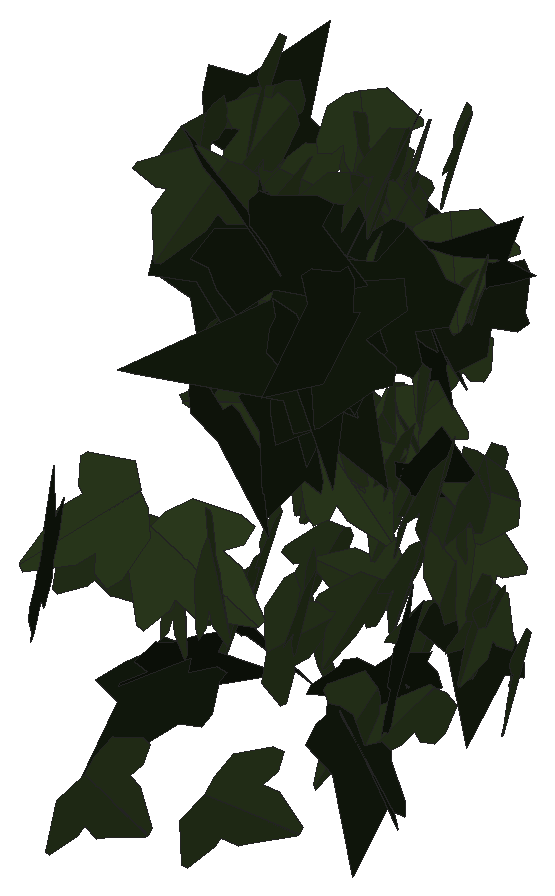
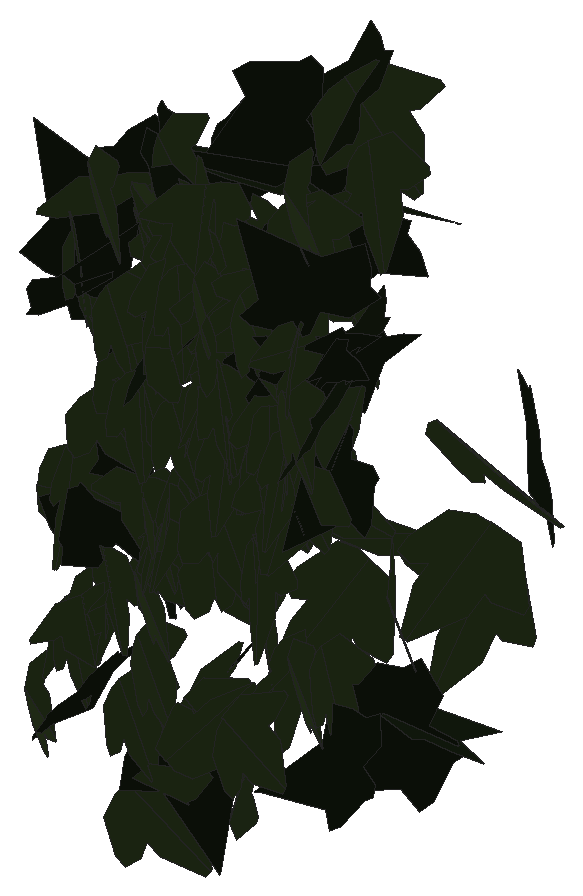
# SketchUp Ruby script. Lengths in inches.
U = 1.inch
M = Sketchup.active_model
def pt(a) = Geom::Point3d.new(a.map { |v| v * U })
def face(e, loops, mat)
  f = e.add_face(loops[0].map { |a| pt(a) })
  loops[1..].each { |l| e.add_face(l.map { |a| pt(a) }).erase! }
  f.material = f.back_material = mat if mat
  f
end
# faces: each face lists its corners as indices into pts; further lists are holes
def faces(e, pts, list, mat = nil) = list.each { |f| face(e, (f[0].is_a?(Array) ? f : [f]).map { |l| l.map { |i| pts[i] } }, mat) }
# xy, xz, yz: faces in a plane at the given z, y or x. An outline is a flat list of corners, or four numbers for a rectangle; further outlines are holes
def ring(l) = l.size == 4 ? [[l[0], l[1]], [l[2], l[1]], [l[2], l[3]], [l[0], l[3]]] : l.each_slice(2).to_a
def flat(e, list, mat, &to3) = list.each { |f| face(e, (f[0].is_a?(Array) ? f : [f]).map { |l| ring(l).map { |u, v| to3.(u, v) } }, mat) }
def xy(e, z, list, mat = nil) = flat(e, list, mat) { |x, y| [x, y, z] }
def xz(e, y, list, mat = nil) = flat(e, list, mat) { |x, z| [x, y, z] }
def yz(e, x, list, mat = nil) = flat(e, list, mat) { |y, z| [x, y, z] }
def lines(e, pts, list) = list.each { |a, b| e.add_line(pt(pts[a]), pt(pts[b])) }
# prism: a flat outline (further loops are holes) pulled along v
def prism(e, loops, v, mat = nil)
  f = face(e, loops, mat); d = Geom::Vector3d.new(v.map { |x| x * U })
  f.pushpull(f.normal.samedirection?(d) ? d.length : -d.length)
end
def box(e, o, s, mat = nil) = prism(e, [[o, [o[0] + s[0], o[1], o[2]], [o[0] + s[0], o[1] + s[1], o[2]], [o[0], o[1] + s[1], o[2]]]], [0, 0, s[2]], mat)
def at(x, y, z, deg = 0) = Geom::Transformation.translation(pt([x, y, z])) * Geom::Transformation.rotation(ORIGIN, Z_AXIS, deg.degrees)
def axes(o, x, y, z) = Geom::Transformation.new([*x, 0, *y, 0, *z, 0, *pt(o).to_a, 1])
def part(name) = M.definitions.add(name)
# library, detail: a bought-in or finely detailed component or shape, given as its bounding box
def library(name, o, s) = part(name).tap { |d| box(d.entities, o, s) }
def detail(e, o, s) = box(e.add_group.entities, o, s)
def put(e, d, t, mat = nil) = e.add_instance(d, t).tap { |i| i.material = mat if mat }
def group(e, t, mat = nil) = e.add_group.tap { |g| g.transformation = t; g.material = mat if mat }.entities
root = M.entities
M.materials.add("efeu1").color = [18, 25, 13]
M.materials.add("efeu2").color = [43, 57, 29]
c1 = part("ivyleaf_9")
p = [[1.54,2.16,1.25],[1.36,2.04,1.19],[-0.21,0.99,0.68],[-0.71,1.11,0.82],[-0.85,0.86,0.67],[-0.8,0.17,0.21],
  [-0.9,-0.01,0.1],[-0.67,-0.16,-0.02],[-0.08,-0.08,-0.05],[-0.03,-0.6,-0.4],[0.65,-0.88,-0.66],[0.83,-0.6,-0.49],
  [1.29,-0.42,-0.43],[1.8125,-0.07,-0.26],[1.21,0.44,0.15]]
faces(c1.entities,p,[[0,1,2,3,4,5,6,7,8,9,10,11,12,13,14]],"efeu1")
c2 = part("ivyleaf_10")
p = [[0,0.5,-0.03],[-0.0625,2.02,-0.43],[-0.19,2.01,-0.46],[-0.54,1.05,-0.29],[-0.52,0.625,-0.18],[-0.83,0.76,-0.28],
  [-1.16,0.64,-0.33],[-1.15,0.33,-0.24],[-0.77,-0.39,0.02],[-0.3,-0.51,0.16],[0.04,-0.48,0.23],[-0.02,2.01,-0.4375],
  [-0.06,2.01,-0.43],[0.04,-0.49,0.23],[0.67,-0.49,0.14],[1.38,0.36,-0.2],[1.375,0.51,-0.24],[0.81,0.65,-0.19],
  [0.62,0.59,-0.15],[0.6,1.09,-0.28],[0.5,1.23,-0.31]]
faces(c2.entities,p,[[0,1,2,3,4,5,6,7,8,9,10],[11,12,0,13,14,15,16,17,18,19,20]],"efeu2")
put(root,c1,axes([511.15,135.28,178.95],[0.14164,0.57002,0.50842],[0.12834,0.49198,-0.58734],[-0.75296,0.19108,-0.00447]))
put(root,c2,axes([511.12,136.73,180.52],[0.21333,-0.6716,0.06352],[0.01506,-0.06187,-0.70465],[0.67443,0.21381,-0.00436]))
put(root,c2,axes([511.75,131.78,177.48],[-0.69811,0.54569,0.46461],[-0.76157,-0.49096,-0.43742],[-0.01149,-0.61349,0.76332]))
put(root,c2,axes([510.92,132.44,176.25],[-0.58613,-0.46292,-0.50371],[0.41735,0.2929,-0.74147],[0.5911,-0.66583,0.02404]))
put(root,c2,axes([511.37,136.4,181.1],[-0.24625,0.52454,-0.45681],[-0.19157,0.4147,0.57947],[0.66867,0.31198,-0.00222]))
put(root,c1,axes([510.75,136.51,180.25],[0.36194,-0.58497,0.07417],[0.04125,-0.06031,-0.70113],[0.63511,0.33728,0.00327]))
put(root,c1,axes([510.93,136.33,182.25],[-0.36547,-0.07879,0.68714],[0.66894,0.15724,0.37382],[-0.17577,0.76224,-0.00609]))
put(root,c1,axes([511.51,130.03,176.5625],[-0.04464,0.21702,0.92704],[-0.11244,0.92036,-0.22087],[-0.94544,-0.11971,-0.0175]))
put(root,c2,axes([511.19,136.21,181.47],[0.03368,-0.16022,0.69276],[-0.1428,0.67788,0.16372],[-0.69656,-0.14672,-0.00007]))
put(root,c2,axes([511.23,136.57,179.05],[-0.58682,-0.40969,-0.16454],[0.14406,0.08102,-0.71552],[0.41733,-0.60405,0.01563]))
put(root,c2,axes([511.34,136.58,179.54],[-0.02157,-0.61766,-0.40572],[0.02782,0.40493,-0.61793],[0.73848,-0.03329,0.01143]))
put(root,c1,axes([510.75,135.53,173.74],[0.62716,-0.26128,0.25886],[0.25675,-0.07778,-0.66174],[0.29319,0.62699,0.02578]))
put(root,c2,axes([511.3125,135.45,179.11],[-0.03052,-0.34319,-0.65587],[0.02977,-0.65646,0.34212],[-0.73963,-0.01226,0.04083]))
put(root,c1,axes([511.09,133.5,173.4375],[0.57098,0.39004,0.50293],[0.37927,0.33619,-0.6813],[-0.5535,0.63272,0.05198]))
put(root,c1,axes([511.34,136.28,181.11],[-0.24178,-0.73558,0.02858],[-0.00916,-0.02707,-0.7743],[0.73608,-0.24196,-0.00025]))
put(root,c2,axes([511.5625,134.11,183.53],[-0.02096,-0.82382,-0.06096],[0.0074,0.06079,-0.82407],[0.82604,-0.02145,0.00583]))
put(root,c2,axes([511.61,135.88,183.32],[-0.2337,-0.68713,0.08115],[-0.01539,-0.08047,-0.72569],[0.69173,-0.23394,0.01127]))
put(root,c1,axes([511.35,135.32,180.48],[-0.15787,-0.84297,0.08874],[-0.01523,-0.08743,-0.85762],[0.84749,-0.1586,0.00112]))
put(root,c2,axes([511.2,136.62,178.95],[0.35062,-0.25449,0.59573],[0.48582,-0.34481,-0.43323],[0.42854,0.59911,0.00372]))
put(root,c1,axes([511.7,133.5,173.54],[-0.85936,-0.26578,-0.23105],[0.35996,-0.43576,-0.69933],[0.10194,-0.70187,0.52168]))
put(root,c2,axes([511.44,136.2,183.875],[0.37854,-0.52663,0.45237],[0.24867,-0.37821,-0.64838],[0.64819,0.45265,-0.01545]))
put(root,c2,axes([511.67,135.89,182.92],[-0.0864,-0.47363,0.62044],[0.0382,-0.62605,-0.47259],[0.77962,-0.02182,0.09191]))
put(root,c2,axes([511.74,136.43,179.79],[0.02039,-0.7307,-0.24751],[-0.02139,0.24696,-0.73085],[0.77118,0.02617,-0.01372]))
put(root,c2,axes([512.26,135.12,178.15],[0.24334,0.0442,-0.83711],[-0.83344,0.10625,-0.23667],[0.08991,0.86527,0.07182]))
put(root,c2,axes([511.65,135.89,175.22],[0.38524,-0.56711,0.15923],[0.07581,-0.14094,-0.6854],[0.58414,0.3923,-0.01606]))
put(root,c2,axes([511.9,136.05,179.77],[0.4714,-0.25713,-0.48283],[-0.2071,0.50605,-0.47168],[0.50631,0.44639,0.25661]))
put(root,c1,axes([511.58,136.21,181.18],[-0.34428,-0.58416,-0.37826],[0.20773,0.31651,-0.67788],[0.66421,-0.40178,0.01595]))
put(root,c2,axes([511.89,135.75,178.76],[-0.1119,-0.7104,0.25282],[-0.04232,-0.24927,-0.71915],[0.75286,-0.1196,-0.00285]))
put(root,c2,axes([511.86,134.84,174.77],[0.12195,-0.76393,0.0114],[-0.00243,-0.01193,-0.77359],[0.76401,0.1219,-0.00428]))
put(root,c2,axes([511.83,136.15,179.89],[-0.24136,-0.64895,-0.38243],[0.18733,0.33725,-0.69051],[0.72958,-0.30128,0.05078]))
put(root,c2,axes([511.96,137.02,174.56],[0.00641,-0.60134,0.43483],[0.03157,-0.43423,-0.60098],[0.74141,0.02369,0.02183]))
put(root,c2,axes([511.99,136.64,181.83],[0.11906,-0.72023,0.14581],[0.00285,-0.14726,-0.72971],[0.73484,0.11726,-0.02079]))
put(root,c2,axes([512.05,136.33,177.28],[0.09519,-0.68907,-0.31051],[-0.035,0.3086,-0.69558],[0.75499,0.10118,0.00691]))
put(root,c2,axes([511.46,133.62,175.38],[0.26575,-0.1273,0.81893],[0.694,-0.4359,-0.29297],[0.453,0.74247,-0.03159]))
put(root,c2,axes([512.37,136.87,180.49],[-0.05394,-0.6894,0.01608],[-0.00223,-0.01596,-0.6915],[0.68958,-0.05397,-0.00098]))
put(root,c2,axes([512.44,136.34,172.89],[-0.51025,0.54537,-0.05767],[-0.0399,0.04165,0.74685],[0.54695,0.51181,0.00068]))
put(root,c2,axes([512,136.18,181.92],[-0.36607,-0.22679,-0.57957],[0.50135,0.29093,-0.43051],[0.36875,-0.62069,0.00997]))
put(root,c2,axes([512.44,136.64,179.4],[-0.10488,-0.6501,-0.24321],[0.05441,0.23752,-0.65834],[0.69197,-0.11721,0.0149]))
put(root,c2,axes([512.76,136.52,177.96],[-0.58484,-0.21196,0.36112],[-0.34121,-0.11833,-0.62205],[0.24271,-0.67709,-0.00433]))
put(root,c2,axes([512.64,136.67,180.51],[0.44296,-0.54735,-0.35738],[-0.16339,0.3253,-0.70073],[0.63295,0.46703,0.06922]))
put(root,c2,axes([512.57,136.16,177.2],[-0.11301,-0.63831,0.27205],[0.03613,-0.28067,-0.64353],[0.69292,-0.08947,0.07793]))
put(root,c2,axes([512.5625,136.75,181.38],[0.02656,-0.66266,0.30431],[0.10081,-0.29825,-0.65827],[0.72219,0.066,0.0807]))
put(root,c1,axes([512.34,133.9375,182.16],[-0.42104,-0.5625,-0.56083],[0.31982,0.46097,-0.70245],[0.72708,-0.5285,-0.01578]))
put(root,c2,axes([512.89,132.81,183.65],[-0.48729,-0.59548,0.47357],[-0.23981,-0.4135,-0.7667],[0.72205,-0.5392,0.06496]))
put(root,c2,axes([512.3,134.9,181.6],[0.64559,0.37467,0.26315],[0.21905,0.14669,-0.74626],[-0.40205,0.68155,0.01596]))
put(root,c2,axes([511.96,132.98,176.3],[-0.38496,-0.59194,-0.69533],[0.95696,-0.32376,-0.19318],[-0.11963,-0.68501,0.69216]))
put(root,c2,axes([512.89,137.13,174.04],[0.0812,0.42894,0.55127],[-0.08327,-0.54508,0.43639],[0.69351,-0.11568,-0.01215]))
put(root,c2,axes([513.13,136.17,176.84],[-0.30585,-0.44508,0.40869],[-0.24407,-0.32803,-0.5399],[0.55276,-0.39111,-0.01226]))
put(root,c2,axes([512.92,134.47,174.19],[0.06677,-0.15338,-0.86122],[0.13976,0.8545,-0.14135],[0.86353,-0.12643,0.08947]))
put(root,c2,axes([512.97,136.58,181.77],[0.31888,-0.67068,0.08663],[0.031,-0.08118,-0.74259],[0.67554,0.32031,-0.00681]))
put(root,c2,axes([512.92,129.66,173.65],[-0.2394,-0.73155,-0.59799],[0.22601,0.55464,-0.769],[0.91743,-0.32753,0.0334]))
put(root,c2,axes([513.35,136.25,179.74],[0.03558,-0.05301,0.75932],[-0.49123,0.57906,0.06344],[-0.58144,-0.49247,-0.00713]))
put(root,c2,axes([513.15,136.51,174.27],[-0.07921,-0.57044,0.38723],[-0.02074,-0.38763,-0.57527],[0.68914,-0.07723,0.0272]))
put(root,c2,axes([513.23,136.92,179.73],[-0.08744,-0.66797,0.14057],[0.0166,-0.14375,-0.6728],[0.6824,-0.0821,0.03437]))
put(root,c2,axes([513.33,136.72,181.88],[-0.01785,-0.71046,-0.12065],[0.01133,0.1204,-0.71063],[0.72054,-0.01949,0.00819]))
put(root,c2,axes([513.16,136.37,183.4],[0.44133,0.54897,0.06696],[0.00352,0.08287,-0.70267],[-0.55303,0.43862,0.04896]))
put(root,c2,axes([513.26,137.24,181.07],[0.03521,-0.27822,0.64107],[0.11882,-0.63015,-0.28001],[0.68866,0.12295,0.01553]))
put(root,c2,axes([513.41,135.9,182.32],[-0.44488,-0.62171,0.01663],[-0.00799,-0.01472,-0.76448],[0.62188,-0.44495,0.00207]))
put(root,c1,axes([512.86,134.06,180.41],[0.58839,-0.58371,-0.01156],[-0.00435,0.01203,-0.82879],[0.58381,0.58838,0.00548]))
put(root,c1,axes([512.86,133.15,179.04],[0.33869,-0.71847,0.40917],[0.22414,-0.34582,-0.79277],[0.79585,0.40315,0.04914]))
put(root,c1,axes([512.84,132.9375,183.73],[0.44794,-0.55382,0.40403],[0.26541,-0.3049,-0.71218],[0.63207,0.52051,0.01272]))
put(root,c2,axes([513.53,134.48,175.46],[0.3406,-0.68731,-0.16805],[-0.05241,0.16149,-0.7667],[0.70562,0.34376,0.02417]))
put(root,c1,axes([513.17,136.3,181.1],[0.07031,-0.75365,0.20487],[0.04045,-0.20191,-0.75663],[0.77995,0.07841,0.02077]))
put(root,c2,axes([513.76,135.34,177.97],[-0.14378,0.1965,0.73988],[-0.41548,0.61227,-0.24335],[-0.64297,-0.43957,-0.0082]))
put(root,c1,axes([513.26,134.4,178.45],[-0.00577,-0.62962,0.49023],[0.02542,-0.49014,-0.6292],[0.79755,0.01107,0.0236]))
put(root,c1,axes([513.85,135.86,173.39],[0.15985,0.64181,-0.39188],[-0.12234,-0.3731,-0.66096],[-0.74197,0.19979,0.02455]))
put(root,c2,axes([513.65,136.56,181.82],[-0.21744,-0.6239,-0.26462],[0.1252,0.23614,-0.65963],[0.66603,-0.24807,0.0376]))
put(root,c2,axes([513.17,136.17,182.82],[0.1606,-0.0401,0.74316],[0.71269,-0.21072,-0.16539],[0.21439,0.73053,-0.00691]))
put(root,c2,axes([514.05,136.75,172.48],[-0.35307,-0.4629,0.51184],[-0.28459,-0.42611,-0.58168],[0.6287,-0.45284,0.02414]))
put(root,c2,axes([513.77,136.21,177.87],[0.10407,-0.63127,-0.43559],[0.0774,0.44598,-0.62784],[0.76305,0.04086,0.1231]))
put(root,c2,axes([513.47,135.41,177.26],[0.4188,0.49834,0.42173],[0.23758,0.35035,-0.64993],[-0.60807,0.48011,0.03652]))
put(root,c2,axes([513.88,136.64,177.66],[-0.53158,0.39674,0.17608],[-0.12755,0.12334,-0.66295],[-0.4149,-0.54623,-0.0218]))
put(root,c2,axes([513.85,136.96,176.45],[0.33264,-0.56594,0.13751],[0.05092,-0.12949,-0.65611],[0.58018,0.33584,-0.02125]))
put(root,c2,axes([513.96,136.76,175.15],[0.17984,-0.69975,0.15182],[0.04068,-0.1463,-0.72248],[0.71487,0.18436,0.00292]))
put(root,c2,axes([513.94,136.45,176.78],[-0.13375,-0.55717,0.40935],[0.15852,-0.43054,-0.53422],[0.67296,-0.00932,0.2072]))
put(root,c2,axes([513.94,135.6875,182.56],[-0.12076,-0.55655,-0.5518],[0.21685,0.51278,-0.56466],[0.75313,-0.23689,0.07411]))
put(root,c1,axes([513.9,134.3,180.64],[-0.54808,-0.38741,-0.45292],[0.40814,0.20444,-0.66876],[0.43433,-0.68098,0.05689]))
put(root,c2,axes([514.32,136.61,180.1],[-0.51682,-0.39888,0.23305],[-0.18575,-0.14075,-0.65284],[0.42297,-0.54919,-0.00195]))
put(root,c2,axes([514.17,136.6875,179.73],[-0.15655,-0.67232,-0.06515],[0.00849,0.06491,-0.69028],[0.67542,-0.15665,-0.00642]))
put(root,c2,axes([514.15,136.3,177.61],[0.23287,-0.71141,0.02055],[0.00641,-0.01952,-0.74856],[0.71168,0.23296,0.00002]))
put(root,c2,axes([514.07,136.7,178.03],[0.66059,0.17652,0.0558],[0.05174,0.02248,-0.68372],[-0.17775,0.66257,0.00833]))
put(root,c2,axes([513.54,133.82,181.1],[0.05611,-0.03226,-0.86542],[0.83204,-0.23853,0.06284],[-0.2402,-0.83379,0.01551]))
put(root,c2,axes([514.125,135.61,182.51],[-0.7121,0.1639,-0.25147],[0.23978,-0.07885,-0.7304],[-0.18057,-0.75107,0.02181]))
put(root,c2,axes([514.34,136.77,174.22],[-0.00983,-0.68823,0.14291],[-0.00744,-0.14281,-0.68828],[0.70287,-0.01114,-0.00528]))
put(root,c2,axes([514.36,136.16,181.18],[0.31151,-0.61086,-0.26841],[-0.06091,0.26895,-0.68278],[0.66445,0.31104,0.06325]))
put(root,c2,axes([514.28,135.99,182.1875],[0.40067,-0.54006,0.30653],[-0.12772,0.28533,0.66965],[-0.60771,-0.41603,0.06136]))
put(root,c1,axes([513.9375,136.47,180.68],[0.53118,-0.5476,0.02157],[0.0117,-0.01871,-0.76288],[0.5479,0.53129,-0.00463]))
put(root,c1,axes([514.28,135.18,181.97],[-0.55929,-0.37036,-0.39864],[0.35211,0.18952,-0.67007],[0.41485,-0.66016,0.03128]))
put(root,c1,axes([513.98,132.53,183.14],[-0.03634,-0.04612,-0.91215],[0.28084,0.86808,-0.05508],[0.86907,-0.28245,-0.02034]))
put(root,c2,axes([514.37,134.85,173.3],[0.01009,-0.38628,0.67921],[0.22162,-0.64996,-0.37293],[0.74928,0.19744,0.10116]))
put(root,c2,axes([514.42,135.65,183.48],[0.13768,-0.65321,0.33663],[0.14846,-0.3107,-0.66361],[0.71969,0.18905,0.07249]))
put(root,c1,axes([514.64,135.53,183.57],[-0.48936,0.42308,-0.43345],[0.33373,-0.27669,-0.64685],[-0.50546,-0.59228,-0.00744]))
put(root,c2,axes([514.7,136.96,179.4],[-0.43661,-0.41397,0.34569],[-0.07898,-0.3909,-0.56786],[0.53351,-0.39665,0.19884]))
put(root,c2,axes([514.65,136.7,181.11],[0.00844,-0.68794,0.11701],[-0.00615,-0.11709,-0.68796],[0.6978,0.00729,-0.00748]))
put(root,c2,axes([514.69,135.94,182.125],[0.45412,-0.56948,-0.07185],[-0.03729,0.06215,-0.72831],[0.57278,0.45555,0.00954]))
put(root,c2,axes([514.76,136.68,176.4],[0.58079,-0.27628,-0.20982],[-0.11968,0.22448,-0.62686],[0.32562,0.57528,0.14384]))
put(root,c2,axes([514.49,135.27,181.41],[-0.18283,-0.34077,-0.73583],[0.47144,0.56905,-0.38067],[0.65978,-0.50105,0.06811]))
put(root,c1,axes([514.27,135.07,172.43],[0.24826,-0.48225,0.58906],[0.26019,-0.52853,-0.54235],[0.71544,0.35956,-0.00716]))
put(root,c2,axes([514.85,135.92,179.3],[0.41892,-0.48326,-0.26997],[-0.093,0.27231,-0.63176],[0.54569,0.4174,0.09958]))
put(root,c2,axes([514.8125,136.93,183.39],[0.35846,-0.60648,0.06114],[0.02468,-0.05643,-0.70446],[0.60906,0.35923,-0.00744]))
put(root,c2,axes([514.71,130.76,173.51],[-0.33828,-0.54157,-0.74252],[0.35638,0.65201,-0.63792],[0.84713,-0.49056,-0.02814]))
put(root,c1,axes([515.15,135.57,180.42],[0.36161,0.02148,-0.6927],[-0.693,0.00382,-0.36165],[-0.00655,0.7814,0.02081]))
put(root,c1,axes([515.87,132.84,181.64],[-1.28529,0.39131,0.38776],[-0.56129,-0.58078,-1.09127],[-0.16035,-1.10363,0.71177]))
put(root,c2,axes([515.18,135.96,175.35],[0.06588,0.27428,-0.67419],[-0.06972,0.67621,0.26829],[0.7245,0.04013,0.08712]))
put(root,c1,axes([514.88,136.43,176.8],[0.73634,0.00783,0.21599],[-0.21605,0.00592,0.73634],[0.00585,-0.76735,0.00788]))
put(root,c1,axes([514.83,133.16,180.625],[0.12528,-0.60232,-0.53817],[-0.02716,0.54115,-0.61198],[0.80726,0.11168,0.06293]))
put(root,c1,axes([514.85,134.3,172.91],[0.07195,-0.77133,0.35049],[0.04062,-0.34821,-0.77464],[0.84625,0.0823,0.00738]))
put(root,c2,axes([514.56,130.55,178.06],[0.1665,-0.09511,0.96969],[0.85871,-0.45051,-0.19163],[0.46039,0.87468,0.00674]))
put(root,c2,axes([515.16,136.875,175.66],[0.28703,0.59829,-0.1598],[-0.0624,-0.14729,-0.66353],[-0.61611,0.29364,-0.00724]))
put(root,c1,axes([515.125,137.03,174.21],[-0.01479,-0.75112,0.18296],[0.01572,-0.18325,-0.75103],[0.77292,-0.01065,0.01877]))
put(root,c1,axes([516.1,133.95,181.46],[-0.23054,0.07388,0.8996],[-0.89308,0.11607,-0.2384],[-0.13099,-0.92139,0.0421]))
put(root,c2,axes([516.03,136.33,177.24],[-0.0112,0.05609,-0.73815],[-0.73524,0.08515,0.01763],[0.08623,0.73331,0.05442]))
put(root,c1,axes([515.95,136.19,180.52],[-0.54258,-0.55871,0.11639],[0.09143,0.07342,0.77868],[-0.56333,0.55004,0.01428]))
put(root,c1,axes([515.25,132.4375,181.38],[0.27524,-0.8008,0.36856],[0.10582,-0.3533,-0.84667],[0.87516,0.29457,-0.01354]))
put(root,c1,axes([515.59,133,181.92],[0.1883,-0.35523,-0.79583],[0.42103,-0.6758,0.40127],[-0.76307,-0.46054,0.02502]))
put(root,c2,axes([515.82,136.32,174.94],[0.07461,-0.70159,0.00059],[-0.00055,-0.00065,-0.70554],[0.70159,0.07461,-0.00061]))
put(root,c2,axes([515.89,135.96,181.37],[0.05768,-0.70058,-0.01657],[-0.00573,0.01616,-0.70294],[0.70075,0.05779,-0.00439]))
put(root,c2,axes([515.91,134.97,178.22],[0.19286,-0.77536,-0.08895],[-0.03156,0.08381,-0.79892],[0.77981,0.19515,-0.01033]))
put(root,c2,axes([515.69,135.57,182.3],[0.4835,0.62664,0.04036],[0.02415,0.03235,-0.79148],[-0.62747,0.4841,0.00064]))
put(root,c2,axes([515.87,136.09,177.53],[0.03192,-0.68244,-0.38392],[0.08026,0.38507,-0.67781],[0.7789,-0.01171,0.08558]))
put(root,c2,axes([515.8,136.43,175.08],[-0.00479,0.48929,-0.55508],[-0.01492,-0.55505,-0.48912],[-0.7398,0.00803,0.01346]))
put(root,c2,axes([515.97,136.02,181.68],[0.36201,-0.59674,-0.17286],[-0.04451,0.17464,-0.69609],[0.61967,0.36115,0.05099]))
put(root,c1,axes([515.5,135.76,181.56],[0.6537,0.41711,-0.05239],[0.04318,0.02971,0.77544],[0.41817,-0.65513,0.00182]))
put(root,c1,axes([515.75,133.9375,174.6],[-0.06359,0.53229,0.76026],[0.07749,-0.75634,0.53602],[0.92484,0.09997,0.00736]))
put(root,c2,axes([515.9,137.15,173.86],[0.31679,-0.43259,0.41337],[0.25143,-0.32819,-0.53613],[0.54294,0.40438,0.00709]))
